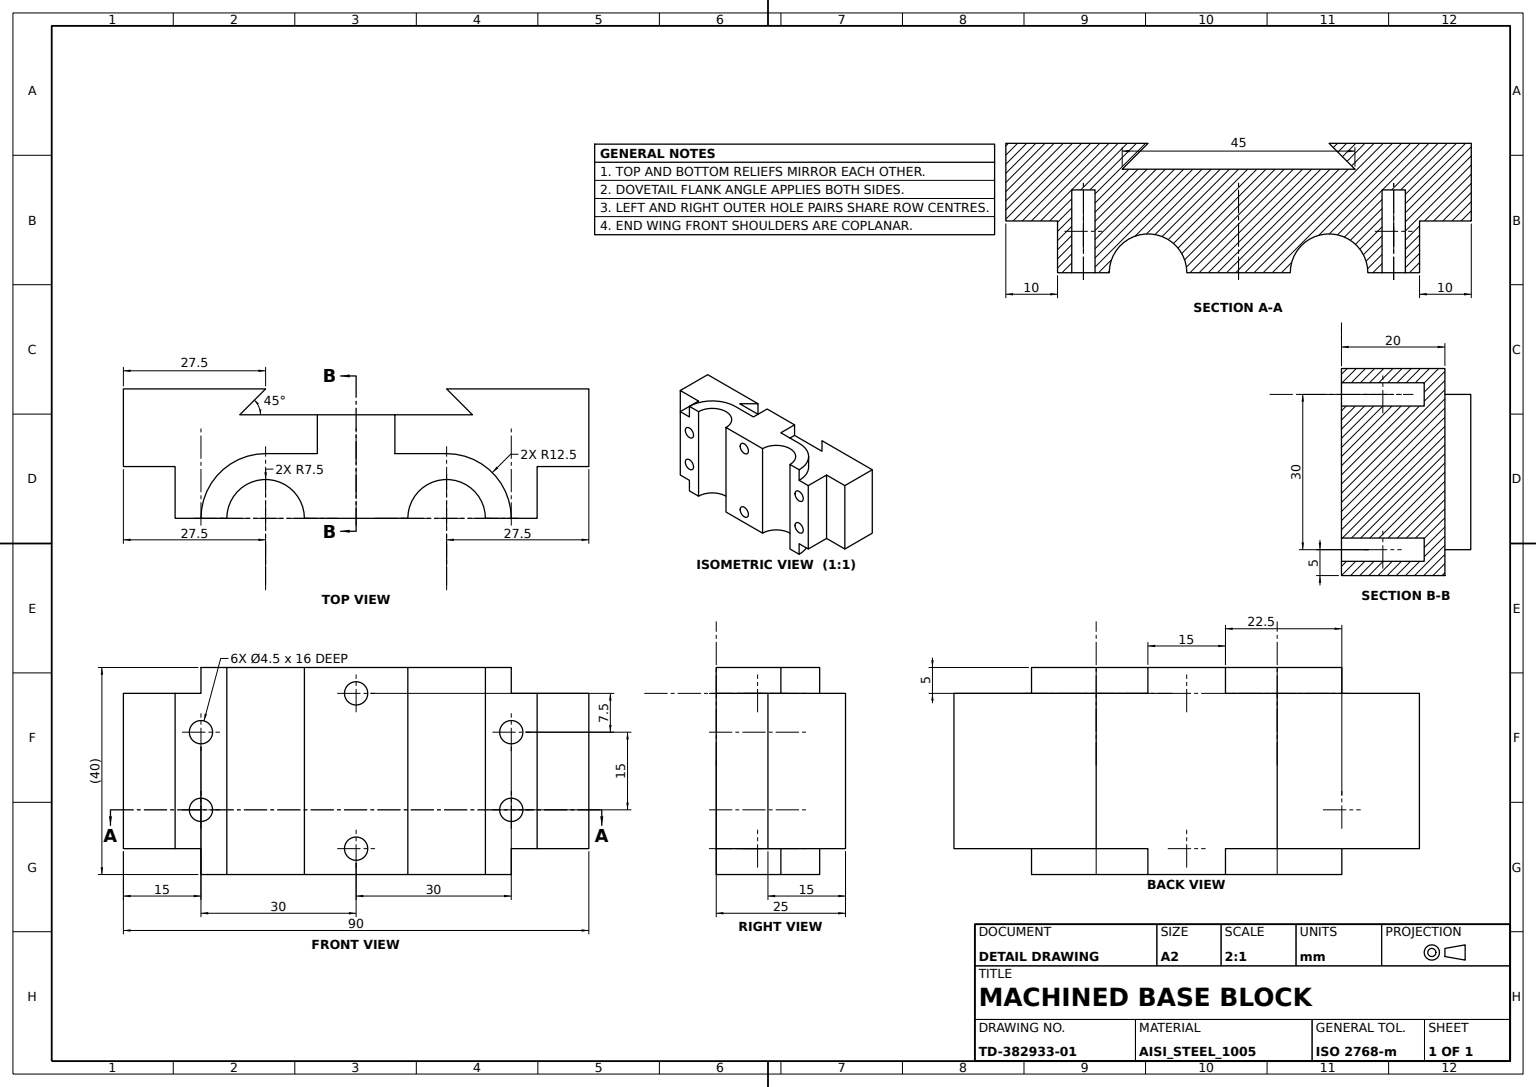
ISO-10303-21;
HEADER;
FILE_DESCRIPTION((''),'2;1');
FILE_NAME('','',(''),(''),'','','');
FILE_SCHEMA(('AUTOMOTIVE_DESIGN'));
ENDSEC;
DATA;
#1=APPLICATION_CONTEXT('');
#2=PRODUCT_CONTEXT('',#1,'mechanical');
#3=PRODUCT('','','',(#2));
#4=PRODUCT_DEFINITION_FORMATION('','',#3);
#5=PRODUCT_DEFINITION_CONTEXT('',#1,'design');
#6=PRODUCT_DEFINITION('','',#4,#5);
#7=PRODUCT_DEFINITION_SHAPE('','',#6);
#8=(LENGTH_UNIT()NAMED_UNIT(*)SI_UNIT(.MILLI.,.METRE.));
#9=(NAMED_UNIT(*)PLANE_ANGLE_UNIT()SI_UNIT($,.RADIAN.));
#10=(NAMED_UNIT(*)SI_UNIT($,.STERADIAN.)SOLID_ANGLE_UNIT());
#11=UNCERTAINTY_MEASURE_WITH_UNIT(LENGTH_MEASURE(0.005),#8,'distance_accuracy_value','');
#12=(GEOMETRIC_REPRESENTATION_CONTEXT(3)GLOBAL_UNCERTAINTY_ASSIGNED_CONTEXT((#11))GLOBAL_UNIT_ASSIGNED_CONTEXT((#8,#9,#10))REPRESENTATION_CONTEXT('',''));
#13=CARTESIAN_POINT('',(-20.,-27.75,-7.5));
#14=VERTEX_POINT('',#13);
#15=CARTESIAN_POINT('',(-20.,-30.,-7.5));
#16=DIRECTION('',(-1.,0.,0.));
#17=DIRECTION('',(0.,1.,0.));
#18=AXIS2_PLACEMENT_3D('',#15,#16,#17);
#19=CIRCLE('',#18,2.25);
#20=EDGE_CURVE('',#14,#14,#19,.T.);
#21=ORIENTED_EDGE('',*,*,#20,.T.);
#22=EDGE_LOOP('',(#21));
#23=FACE_BOUND('',#22,.T.);
#24=CARTESIAN_POINT('',(-4.,-27.75,-7.5));
#25=VERTEX_POINT('',#24);
#26=CARTESIAN_POINT('',(-4.,-30.,-7.5));
#27=AXIS2_PLACEMENT_3D('',#26,#16,#17);
#28=CIRCLE('',#27,2.25);
#29=EDGE_CURVE('',#25,#25,#28,.F.);
#30=ORIENTED_EDGE('',*,*,#29,.T.);
#31=EDGE_LOOP('',(#30));
#32=FACE_BOUND('',#31,.T.);
#33=DIRECTION('',(0.,0.,1.));
#34=AXIS2_PLACEMENT_3D('',#26,#16,#33);
#35=CYLINDRICAL_SURFACE('',#34,2.25);
#36=ADVANCED_FACE('',(#23,#32),#35,.F.);
#37=CARTESIAN_POINT('',(-4.,2.25,-15.));
#38=VERTEX_POINT('',#37);
#39=CARTESIAN_POINT('',(-4.,0.,-15.));
#40=AXIS2_PLACEMENT_3D('',#39,#16,#17);
#41=CIRCLE('',#40,2.25);
#42=EDGE_CURVE('',#38,#38,#41,.F.);
#43=ORIENTED_EDGE('',*,*,#42,.F.);
#44=EDGE_LOOP('',(#43));
#45=FACE_BOUND('',#44,.T.);
#46=AXIS2_PLACEMENT_3D('',#39,#16,#33);
#47=PLANE('',#46);
#48=ADVANCED_FACE('',(#45),#47,.T.);
#49=CARTESIAN_POINT('',(5.,17.5,15.));
#50=VERTEX_POINT('',#49);
#51=CARTESIAN_POINT('',(5.,17.5,-15.));
#52=VERTEX_POINT('',#51);
#53=DIRECTION('',(0.,0.,-1.));
#54=VECTOR('',#53,1000.);
#55=LINE('',#49,#54);
#56=EDGE_CURVE('',#50,#52,#55,.T.);
#57=ORIENTED_EDGE('',*,*,#56,.F.);
#58=CARTESIAN_POINT('',(0.,22.5,15.));
#59=VERTEX_POINT('',#58);
#60=DIRECTION('',(0.707106781,-0.707106781,0.));
#61=VECTOR('',#60,1000.);
#62=LINE('',#58,#61);
#63=EDGE_CURVE('',#59,#50,#62,.T.);
#64=ORIENTED_EDGE('',*,*,#63,.F.);
#65=CARTESIAN_POINT('',(0.,22.5,-15.));
#66=VERTEX_POINT('',#65);
#67=LINE('',#58,#54);
#68=EDGE_CURVE('',#59,#66,#67,.T.);
#69=ORIENTED_EDGE('',*,*,#68,.T.);
#70=LINE('',#65,#61);
#71=EDGE_CURVE('',#66,#52,#70,.T.);
#72=ORIENTED_EDGE('',*,*,#71,.T.);
#73=EDGE_LOOP('',(#57,#64,#69,#72));
#74=FACE_BOUND('',#73,.T.);
#75=DIRECTION('',(0.707106781,0.707106781,0.));
#76=DIRECTION('',(-0.707106781,0.707106781,0.));
#77=AXIS2_PLACEMENT_3D('',#58,#75,#76);
#78=PLANE('',#77);
#79=ADVANCED_FACE('',(#74),#78,.F.);
#80=CARTESIAN_POINT('',(-20.,2.25,-15.));
#81=VERTEX_POINT('',#80);
#82=CARTESIAN_POINT('',(-20.,0.,-15.));
#83=AXIS2_PLACEMENT_3D('',#82,#16,#17);
#84=CIRCLE('',#83,2.25);
#85=EDGE_CURVE('',#81,#81,#84,.T.);
#86=ORIENTED_EDGE('',*,*,#85,.T.);
#87=EDGE_LOOP('',(#86));
#88=FACE_BOUND('',#87,.T.);
#89=ORIENTED_EDGE('',*,*,#42,.T.);
#90=EDGE_LOOP('',(#89));
#91=FACE_BOUND('',#90,.T.);
#92=CYLINDRICAL_SURFACE('',#46,2.25);
#93=ADVANCED_FACE('',(#88,#91),#92,.F.);
#94=CARTESIAN_POINT('',(-4.,2.25,15.));
#95=VERTEX_POINT('',#94);
#96=CARTESIAN_POINT('',(-4.,0.,15.));
#97=AXIS2_PLACEMENT_3D('',#96,#16,#17);
#98=CIRCLE('',#97,2.25);
#99=EDGE_CURVE('',#95,#95,#98,.F.);
#100=ORIENTED_EDGE('',*,*,#99,.F.);
#101=EDGE_LOOP('',(#100));
#102=FACE_BOUND('',#101,.T.);
#103=AXIS2_PLACEMENT_3D('',#96,#16,#33);
#104=PLANE('',#103);
#105=ADVANCED_FACE('',(#102),#104,.T.);
#106=CARTESIAN_POINT('',(-20.,27.75,7.5));
#107=VERTEX_POINT('',#106);
#108=CARTESIAN_POINT('',(-20.,30.,7.5));
#109=DIRECTION('',(0.,-1.,0.));
#110=AXIS2_PLACEMENT_3D('',#108,#16,#109);
#111=CIRCLE('',#110,2.25);
#112=EDGE_CURVE('',#107,#107,#111,.T.);
#113=ORIENTED_EDGE('',*,*,#112,.T.);
#114=EDGE_LOOP('',(#113));
#115=FACE_BOUND('',#114,.T.);
#116=CARTESIAN_POINT('',(-4.,27.75,7.5));
#117=VERTEX_POINT('',#116);
#118=CARTESIAN_POINT('',(-4.,30.,7.5));
#119=AXIS2_PLACEMENT_3D('',#118,#16,#109);
#120=CIRCLE('',#119,2.25);
#121=EDGE_CURVE('',#117,#117,#120,.F.);
#122=ORIENTED_EDGE('',*,*,#121,.T.);
#123=EDGE_LOOP('',(#122));
#124=FACE_BOUND('',#123,.T.);
#125=AXIS2_PLACEMENT_3D('',#118,#16,#33);
#126=CYLINDRICAL_SURFACE('',#125,2.25);
#127=ADVANCED_FACE('',(#115,#124),#126,.F.);
#128=CARTESIAN_POINT('',(-20.,2.25,15.));
#129=VERTEX_POINT('',#128);
#130=CARTESIAN_POINT('',(-20.,0.,15.));
#131=AXIS2_PLACEMENT_3D('',#130,#16,#17);
#132=CIRCLE('',#131,2.25);
#133=EDGE_CURVE('',#129,#129,#132,.T.);
#134=ORIENTED_EDGE('',*,*,#133,.F.);
#135=EDGE_LOOP('',(#134));
#136=FACE_BOUND('',#135,.T.);
#137=ORIENTED_EDGE('',*,*,#85,.F.);
#138=EDGE_LOOP('',(#137));
#139=FACE_BOUND('',#138,.T.);
#140=CARTESIAN_POINT('',(-20.,10.,20.));
#141=VERTEX_POINT('',#140);
#142=CARTESIAN_POINT('',(-20.,10.,-20.));
#143=VERTEX_POINT('',#142);
#144=LINE('',#140,#54);
#145=EDGE_CURVE('',#141,#143,#144,.T.);
#146=ORIENTED_EDGE('',*,*,#145,.T.);
#147=CARTESIAN_POINT('',(-20.,-10.,-20.));
#148=VERTEX_POINT('',#147);
#149=VECTOR('',#109,1000.);
#150=LINE('',#142,#149);
#151=EDGE_CURVE('',#143,#148,#150,.T.);
#152=ORIENTED_EDGE('',*,*,#151,.T.);
#153=CARTESIAN_POINT('',(-20.,-10.,20.));
#154=VERTEX_POINT('',#153);
#155=LINE('',#153,#54);
#156=EDGE_CURVE('',#154,#148,#155,.T.);
#157=ORIENTED_EDGE('',*,*,#156,.F.);
#158=LINE('',#140,#149);
#159=EDGE_CURVE('',#141,#154,#158,.T.);
#160=ORIENTED_EDGE('',*,*,#159,.F.);
#161=EDGE_LOOP('',(#146,#152,#157,#160));
#162=FACE_BOUND('',#161,.T.);
#163=DIRECTION('',(1.,0.,0.));
#164=AXIS2_PLACEMENT_3D('',#140,#163,#53);
#165=PLANE('',#164);
#166=ADVANCED_FACE('',(#136,#139,#162),#165,.F.);
#167=CARTESIAN_POINT('',(5.,-17.5,-15.));
#168=VERTEX_POINT('',#167);
#169=CARTESIAN_POINT('',(0.,-22.5,-15.));
#170=VERTEX_POINT('',#169);
#171=DIRECTION('',(-0.707106781,-0.707106781,0.));
#172=VECTOR('',#171,1000.);
#173=LINE('',#167,#172);
#174=EDGE_CURVE('',#168,#170,#173,.T.);
#175=ORIENTED_EDGE('',*,*,#174,.T.);
#176=CARTESIAN_POINT('',(0.,-22.5,15.));
#177=VERTEX_POINT('',#176);
#178=LINE('',#176,#54);
#179=EDGE_CURVE('',#177,#170,#178,.T.);
#180=ORIENTED_EDGE('',*,*,#179,.F.);
#181=CARTESIAN_POINT('',(5.,-17.5,15.));
#182=VERTEX_POINT('',#181);
#183=LINE('',#181,#172);
#184=EDGE_CURVE('',#182,#177,#183,.T.);
#185=ORIENTED_EDGE('',*,*,#184,.F.);
#186=LINE('',#181,#54);
#187=EDGE_CURVE('',#182,#168,#186,.T.);
#188=ORIENTED_EDGE('',*,*,#187,.T.);
#189=EDGE_LOOP('',(#175,#180,#185,#188));
#190=FACE_BOUND('',#189,.T.);
#191=AXIS2_PLACEMENT_3D('',#181,#60,#75);
#192=PLANE('',#191);
#193=ADVANCED_FACE('',(#190),#192,.F.);
#194=CARTESIAN_POINT('',(-20.,-30.,15.));
#195=VERTEX_POINT('',#194);
#196=CARTESIAN_POINT('',(-20.,-35.,15.));
#197=VERTEX_POINT('',#196);
#198=LINE('',#194,#149);
#199=EDGE_CURVE('',#195,#197,#198,.T.);
#200=ORIENTED_EDGE('',*,*,#199,.T.);
#201=CARTESIAN_POINT('',(-10.,-35.,15.));
#202=VERTEX_POINT('',#201);
#203=VECTOR('',#163,1000.);
#204=LINE('',#196,#203);
#205=EDGE_CURVE('',#197,#202,#204,.T.);
#206=ORIENTED_EDGE('',*,*,#205,.T.);
#207=CARTESIAN_POINT('',(-10.,-45.,15.));
#208=VERTEX_POINT('',#207);
#209=LINE('',#201,#149);
#210=EDGE_CURVE('',#202,#208,#209,.T.);
#211=ORIENTED_EDGE('',*,*,#210,.T.);
#212=CARTESIAN_POINT('',(5.,-45.,15.));
#213=VERTEX_POINT('',#212);
#214=LINE('',#207,#203);
#215=EDGE_CURVE('',#208,#213,#214,.T.);
#216=ORIENTED_EDGE('',*,*,#215,.T.);
#217=VECTOR('',#17,1000.);
#218=LINE('',#212,#217);
#219=EDGE_CURVE('',#213,#182,#218,.T.);
#220=ORIENTED_EDGE('',*,*,#219,.T.);
#221=ORIENTED_EDGE('',*,*,#184,.T.);
#222=CARTESIAN_POINT('',(0.,-7.5,15.));
#223=VERTEX_POINT('',#222);
#224=LINE('',#176,#217);
#225=EDGE_CURVE('',#177,#223,#224,.T.);
#226=ORIENTED_EDGE('',*,*,#225,.T.);
#227=CARTESIAN_POINT('',(-7.5,-7.5,15.));
#228=VERTEX_POINT('',#227);
#229=VECTOR('',#16,1000.);
#230=LINE('',#222,#229);
#231=EDGE_CURVE('',#223,#228,#230,.T.);
#232=ORIENTED_EDGE('',*,*,#231,.T.);
#233=CARTESIAN_POINT('',(-7.5,-17.5,15.));
#234=VERTEX_POINT('',#233);
#235=LINE('',#227,#149);
#236=EDGE_CURVE('',#228,#234,#235,.T.);
#237=ORIENTED_EDGE('',*,*,#236,.T.);
#238=CARTESIAN_POINT('',(-20.,-17.5,15.));
#239=AXIS2_PLACEMENT_3D('',#238,#53,#17);
#240=CIRCLE('',#239,12.5);
#241=EDGE_CURVE('',#234,#195,#240,.T.);
#242=ORIENTED_EDGE('',*,*,#241,.T.);
#243=EDGE_LOOP('',(#200,#206,#211,#216,#220,#221,#226,#232,#237,#242));
#244=FACE_BOUND('',#243,.T.);
#245=AXIS2_PLACEMENT_3D('',#238,#53,#16);
#246=PLANE('',#245);
#247=ADVANCED_FACE('',(#244),#246,.F.);
#248=CARTESIAN_POINT('',(-7.5,-17.5,20.));
#249=VERTEX_POINT('',#248);
#250=LINE('',#248,#54);
#251=EDGE_CURVE('',#249,#234,#250,.T.);
#252=ORIENTED_EDGE('',*,*,#251,.F.);
#253=CARTESIAN_POINT('',(-20.,-30.,20.));
#254=VERTEX_POINT('',#253);
#255=CARTESIAN_POINT('',(-20.,-17.5,20.));
#256=AXIS2_PLACEMENT_3D('',#255,#33,#17);
#257=CIRCLE('',#256,12.5);
#258=EDGE_CURVE('',#254,#249,#257,.T.);
#259=ORIENTED_EDGE('',*,*,#258,.F.);
#260=LINE('',#253,#54);
#261=EDGE_CURVE('',#254,#195,#260,.T.);
#262=ORIENTED_EDGE('',*,*,#261,.T.);
#263=ORIENTED_EDGE('',*,*,#241,.F.);
#264=EDGE_LOOP('',(#252,#259,#262,#263));
#265=FACE_BOUND('',#264,.T.);
#266=AXIS2_PLACEMENT_3D('',#255,#53,#16);
#267=CYLINDRICAL_SURFACE('',#266,12.5);
#268=ADVANCED_FACE('',(#265),#267,.T.);
#269=CARTESIAN_POINT('',(-10.,45.,15.));
#270=VERTEX_POINT('',#269);
#271=CARTESIAN_POINT('',(-10.,35.,15.));
#272=VERTEX_POINT('',#271);
#273=LINE('',#269,#149);
#274=EDGE_CURVE('',#270,#272,#273,.T.);
#275=ORIENTED_EDGE('',*,*,#274,.T.);
#276=CARTESIAN_POINT('',(-20.,35.,15.));
#277=VERTEX_POINT('',#276);
#278=LINE('',#271,#229);
#279=EDGE_CURVE('',#272,#277,#278,.T.);
#280=ORIENTED_EDGE('',*,*,#279,.T.);
#281=CARTESIAN_POINT('',(-20.,30.,15.));
#282=VERTEX_POINT('',#281);
#283=LINE('',#276,#149);
#284=EDGE_CURVE('',#277,#282,#283,.T.);
#285=ORIENTED_EDGE('',*,*,#284,.T.);
#286=CARTESIAN_POINT('',(-7.5,17.5,15.));
#287=VERTEX_POINT('',#286);
#288=CARTESIAN_POINT('',(-20.,17.5,15.));
#289=AXIS2_PLACEMENT_3D('',#288,#53,#109);
#290=CIRCLE('',#289,12.5);
#291=EDGE_CURVE('',#282,#287,#290,.T.);
#292=ORIENTED_EDGE('',*,*,#291,.T.);
#293=CARTESIAN_POINT('',(-7.5,7.5,15.));
#294=VERTEX_POINT('',#293);
#295=LINE('',#286,#149);
#296=EDGE_CURVE('',#287,#294,#295,.T.);
#297=ORIENTED_EDGE('',*,*,#296,.T.);
#298=CARTESIAN_POINT('',(0.,7.5,15.));
#299=VERTEX_POINT('',#298);
#300=LINE('',#293,#203);
#301=EDGE_CURVE('',#294,#299,#300,.T.);
#302=ORIENTED_EDGE('',*,*,#301,.T.);
#303=LINE('',#298,#217);
#304=EDGE_CURVE('',#299,#59,#303,.T.);
#305=ORIENTED_EDGE('',*,*,#304,.T.);
#306=ORIENTED_EDGE('',*,*,#63,.T.);
#307=CARTESIAN_POINT('',(5.,45.,15.));
#308=VERTEX_POINT('',#307);
#309=LINE('',#49,#217);
#310=EDGE_CURVE('',#50,#308,#309,.T.);
#311=ORIENTED_EDGE('',*,*,#310,.T.);
#312=LINE('',#307,#229);
#313=EDGE_CURVE('',#308,#270,#312,.T.);
#314=ORIENTED_EDGE('',*,*,#313,.T.);
#315=EDGE_LOOP('',(#275,#280,#285,#292,#297,#302,#305,#306,#311,#314));
#316=FACE_BOUND('',#315,.T.);
#317=AXIS2_PLACEMENT_3D('',#288,#53,#16);
#318=PLANE('',#317);
#319=ADVANCED_FACE('',(#316),#318,.F.);
#320=CARTESIAN_POINT('',(0.,-7.5,-15.));
#321=VERTEX_POINT('',#320);
#322=CARTESIAN_POINT('',(-7.5,-7.5,-15.));
#323=VERTEX_POINT('',#322);
#324=LINE('',#320,#229);
#325=EDGE_CURVE('',#321,#323,#324,.T.);
#326=ORIENTED_EDGE('',*,*,#325,.T.);
#327=CARTESIAN_POINT('',(-7.5,-7.5,-20.));
#328=VERTEX_POINT('',#327);
#329=CARTESIAN_POINT('',(-7.5,-7.5,20.));
#330=LINE('',#329,#54);
#331=EDGE_CURVE('',#323,#328,#330,.T.);
#332=ORIENTED_EDGE('',*,*,#331,.T.);
#333=CARTESIAN_POINT('',(0.,-7.5,-20.));
#334=VERTEX_POINT('',#333);
#335=LINE('',#327,#203);
#336=EDGE_CURVE('',#328,#334,#335,.T.);
#337=ORIENTED_EDGE('',*,*,#336,.T.);
#338=CARTESIAN_POINT('',(0.,-7.5,20.));
#339=LINE('',#338,#54);
#340=EDGE_CURVE('',#321,#334,#339,.T.);
#341=ORIENTED_EDGE('',*,*,#340,.F.);
#342=EDGE_LOOP('',(#326,#332,#337,#341));
#343=FACE_BOUND('',#342,.T.);
#344=AXIS2_PLACEMENT_3D('',#329,#17,#16);
#345=PLANE('',#344);
#346=ADVANCED_FACE('',(#343),#345,.F.);
#347=CARTESIAN_POINT('',(-20.,27.75,-7.5));
#348=VERTEX_POINT('',#347);
#349=CARTESIAN_POINT('',(-20.,30.,-7.5));
#350=AXIS2_PLACEMENT_3D('',#349,#16,#109);
#351=CIRCLE('',#350,2.25);
#352=EDGE_CURVE('',#348,#348,#351,.T.);
#353=ORIENTED_EDGE('',*,*,#352,.F.);
#354=EDGE_LOOP('',(#353));
#355=FACE_BOUND('',#354,.T.);
#356=ORIENTED_EDGE('',*,*,#284,.F.);
#357=CARTESIAN_POINT('',(-20.,35.,-15.));
#358=VERTEX_POINT('',#357);
#359=LINE('',#276,#54);
#360=EDGE_CURVE('',#277,#358,#359,.T.);
#361=ORIENTED_EDGE('',*,*,#360,.T.);
#362=CARTESIAN_POINT('',(-20.,30.,-15.));
#363=VERTEX_POINT('',#362);
#364=LINE('',#357,#149);
#365=EDGE_CURVE('',#358,#363,#364,.T.);
#366=ORIENTED_EDGE('',*,*,#365,.T.);
#367=CARTESIAN_POINT('',(-20.,30.,-20.));
#368=VERTEX_POINT('',#367);
#369=CARTESIAN_POINT('',(-20.,30.,20.));
#370=LINE('',#369,#54);
#371=EDGE_CURVE('',#363,#368,#370,.T.);
#372=ORIENTED_EDGE('',*,*,#371,.T.);
#373=CARTESIAN_POINT('',(-20.,25.,-20.));
#374=VERTEX_POINT('',#373);
#375=LINE('',#367,#149);
#376=EDGE_CURVE('',#368,#374,#375,.T.);
#377=ORIENTED_EDGE('',*,*,#376,.T.);
#378=CARTESIAN_POINT('',(-20.,25.,20.));
#379=VERTEX_POINT('',#378);
#380=LINE('',#378,#54);
#381=EDGE_CURVE('',#379,#374,#380,.T.);
#382=ORIENTED_EDGE('',*,*,#381,.F.);
#383=VERTEX_POINT('',#369);
#384=LINE('',#369,#149);
#385=EDGE_CURVE('',#383,#379,#384,.T.);
#386=ORIENTED_EDGE('',*,*,#385,.F.);
#387=EDGE_CURVE('',#383,#282,#370,.T.);
#388=ORIENTED_EDGE('',*,*,#387,.T.);
#389=EDGE_LOOP('',(#356,#361,#366,#372,#377,#382,#386,#388));
#390=FACE_BOUND('',#389,.T.);
#391=ORIENTED_EDGE('',*,*,#112,.F.);
#392=EDGE_LOOP('',(#391));
#393=FACE_BOUND('',#392,.T.);
#394=AXIS2_PLACEMENT_3D('',#369,#163,#53);
#395=PLANE('',#394);
#396=ADVANCED_FACE('',(#355,#390,#393),#395,.F.);
#397=CARTESIAN_POINT('',(-20.,-25.,-20.));
#398=VERTEX_POINT('',#397);
#399=CARTESIAN_POINT('',(-20.,-17.5,-20.));
#400=AXIS2_PLACEMENT_3D('',#399,#53,#17);
#401=CIRCLE('',#400,7.5);
#402=EDGE_CURVE('',#148,#398,#401,.T.);
#403=ORIENTED_EDGE('',*,*,#402,.T.);
#404=CARTESIAN_POINT('',(-20.,-25.,20.));
#405=VERTEX_POINT('',#404);
#406=LINE('',#404,#54);
#407=EDGE_CURVE('',#405,#398,#406,.T.);
#408=ORIENTED_EDGE('',*,*,#407,.F.);
#409=AXIS2_PLACEMENT_3D('',#255,#53,#17);
#410=CIRCLE('',#409,7.5);
#411=EDGE_CURVE('',#154,#405,#410,.T.);
#412=ORIENTED_EDGE('',*,*,#411,.F.);
#413=ORIENTED_EDGE('',*,*,#156,.T.);
#414=EDGE_LOOP('',(#403,#408,#412,#413));
#415=FACE_BOUND('',#414,.T.);
#416=CYLINDRICAL_SURFACE('',#266,7.5);
#417=ADVANCED_FACE('',(#415),#416,.F.);
#418=CARTESIAN_POINT('',(-4.,-27.75,7.5));
#419=VERTEX_POINT('',#418);
#420=CARTESIAN_POINT('',(-4.,-30.,7.5));
#421=AXIS2_PLACEMENT_3D('',#420,#16,#17);
#422=CIRCLE('',#421,2.25);
#423=EDGE_CURVE('',#419,#419,#422,.F.);
#424=ORIENTED_EDGE('',*,*,#423,.F.);
#425=EDGE_LOOP('',(#424));
#426=FACE_BOUND('',#425,.T.);
#427=AXIS2_PLACEMENT_3D('',#420,#16,#33);
#428=PLANE('',#427);
#429=ADVANCED_FACE('',(#426),#428,.T.);
#430=CARTESIAN_POINT('',(-7.5,7.5,20.));
#431=VERTEX_POINT('',#430);
#432=LINE('',#430,#54);
#433=EDGE_CURVE('',#431,#294,#432,.T.);
#434=ORIENTED_EDGE('',*,*,#433,.T.);
#435=ORIENTED_EDGE('',*,*,#296,.F.);
#436=CARTESIAN_POINT('',(-7.5,17.5,20.));
#437=VERTEX_POINT('',#436);
#438=LINE('',#436,#54);
#439=EDGE_CURVE('',#437,#287,#438,.T.);
#440=ORIENTED_EDGE('',*,*,#439,.F.);
#441=LINE('',#430,#217);
#442=EDGE_CURVE('',#431,#437,#441,.T.);
#443=ORIENTED_EDGE('',*,*,#442,.F.);
#444=EDGE_LOOP('',(#434,#435,#440,#443));
#445=FACE_BOUND('',#444,.T.);
#446=AXIS2_PLACEMENT_3D('',#430,#16,#109);
#447=PLANE('',#446);
#448=ADVANCED_FACE('',(#445),#447,.F.);
#449=CARTESIAN_POINT('',(-10.,-35.,-15.));
#450=VERTEX_POINT('',#449);
#451=LINE('',#201,#54);
#452=EDGE_CURVE('',#202,#450,#451,.T.);
#453=ORIENTED_EDGE('',*,*,#452,.F.);
#454=ORIENTED_EDGE('',*,*,#205,.F.);
#455=CARTESIAN_POINT('',(-20.,-35.,-15.));
#456=VERTEX_POINT('',#455);
#457=LINE('',#196,#54);
#458=EDGE_CURVE('',#197,#456,#457,.T.);
#459=ORIENTED_EDGE('',*,*,#458,.T.);
#460=LINE('',#455,#203);
#461=EDGE_CURVE('',#456,#450,#460,.T.);
#462=ORIENTED_EDGE('',*,*,#461,.T.);
#463=EDGE_LOOP('',(#453,#454,#459,#462));
#464=FACE_BOUND('',#463,.T.);
#465=AXIS2_PLACEMENT_3D('',#196,#17,#33);
#466=PLANE('',#465);
#467=ADVANCED_FACE('',(#464),#466,.F.);
#468=CARTESIAN_POINT('',(0.,7.5,-15.));
#469=VERTEX_POINT('',#468);
#470=LINE('',#468,#217);
#471=EDGE_CURVE('',#469,#66,#470,.T.);
#472=ORIENTED_EDGE('',*,*,#471,.T.);
#473=ORIENTED_EDGE('',*,*,#68,.F.);
#474=ORIENTED_EDGE('',*,*,#304,.F.);
#475=CARTESIAN_POINT('',(0.,7.5,20.));
#476=VERTEX_POINT('',#475);
#477=LINE('',#475,#54);
#478=EDGE_CURVE('',#476,#299,#477,.T.);
#479=ORIENTED_EDGE('',*,*,#478,.F.);
#480=VERTEX_POINT('',#338);
#481=LINE('',#338,#217);
#482=EDGE_CURVE('',#480,#476,#481,.T.);
#483=ORIENTED_EDGE('',*,*,#482,.F.);
#484=EDGE_CURVE('',#480,#223,#339,.T.);
#485=ORIENTED_EDGE('',*,*,#484,.T.);
#486=ORIENTED_EDGE('',*,*,#225,.F.);
#487=ORIENTED_EDGE('',*,*,#179,.T.);
#488=LINE('',#169,#217);
#489=EDGE_CURVE('',#170,#321,#488,.T.);
#490=ORIENTED_EDGE('',*,*,#489,.T.);
#491=ORIENTED_EDGE('',*,*,#340,.T.);
#492=CARTESIAN_POINT('',(0.,7.5,-20.));
#493=VERTEX_POINT('',#492);
#494=LINE('',#333,#217);
#495=EDGE_CURVE('',#334,#493,#494,.T.);
#496=ORIENTED_EDGE('',*,*,#495,.T.);
#497=EDGE_CURVE('',#469,#493,#477,.T.);
#498=ORIENTED_EDGE('',*,*,#497,.F.);
#499=EDGE_LOOP('',(#472,#473,#474,#479,#483,#485,#486,#487,#490,#491,#496,#498));
#500=FACE_BOUND('',#499,.T.);
#501=AXIS2_PLACEMENT_3D('',#338,#16,#33);
#502=PLANE('',#501);
#503=ADVANCED_FACE('',(#500),#502,.F.);
#504=CARTESIAN_POINT('',(-20.,-27.75,7.5));
#505=VERTEX_POINT('',#504);
#506=CARTESIAN_POINT('',(-20.,-30.,7.5));
#507=AXIS2_PLACEMENT_3D('',#506,#16,#17);
#508=CIRCLE('',#507,2.25);
#509=EDGE_CURVE('',#505,#505,#508,.T.);
#510=ORIENTED_EDGE('',*,*,#509,.T.);
#511=EDGE_LOOP('',(#510));
#512=FACE_BOUND('',#511,.T.);
#513=ORIENTED_EDGE('',*,*,#423,.T.);
#514=EDGE_LOOP('',(#513));
#515=FACE_BOUND('',#514,.T.);
#516=CYLINDRICAL_SURFACE('',#427,2.25);
#517=ADVANCED_FACE('',(#512,#515),#516,.F.);
#518=CARTESIAN_POINT('',(-4.,27.75,-7.5));
#519=VERTEX_POINT('',#518);
#520=CARTESIAN_POINT('',(-4.,30.,-7.5));
#521=AXIS2_PLACEMENT_3D('',#520,#16,#109);
#522=CIRCLE('',#521,2.25);
#523=EDGE_CURVE('',#519,#519,#522,.F.);
#524=ORIENTED_EDGE('',*,*,#523,.T.);
#525=EDGE_LOOP('',(#524));
#526=FACE_BOUND('',#525,.T.);
#527=ORIENTED_EDGE('',*,*,#352,.T.);
#528=EDGE_LOOP('',(#527));
#529=FACE_BOUND('',#528,.T.);
#530=AXIS2_PLACEMENT_3D('',#520,#16,#33);
#531=CYLINDRICAL_SURFACE('',#530,2.25);
#532=ADVANCED_FACE('',(#526,#529),#531,.F.);
#533=ORIENTED_EDGE('',*,*,#325,.F.);
#534=ORIENTED_EDGE('',*,*,#489,.F.);
#535=ORIENTED_EDGE('',*,*,#174,.F.);
#536=CARTESIAN_POINT('',(5.,-45.,-15.));
#537=VERTEX_POINT('',#536);
#538=LINE('',#536,#217);
#539=EDGE_CURVE('',#537,#168,#538,.T.);
#540=ORIENTED_EDGE('',*,*,#539,.F.);
#541=CARTESIAN_POINT('',(-10.,-45.,-15.));
#542=VERTEX_POINT('',#541);
#543=LINE('',#541,#203);
#544=EDGE_CURVE('',#542,#537,#543,.T.);
#545=ORIENTED_EDGE('',*,*,#544,.F.);
#546=LINE('',#449,#149);
#547=EDGE_CURVE('',#450,#542,#546,.T.);
#548=ORIENTED_EDGE('',*,*,#547,.F.);
#549=ORIENTED_EDGE('',*,*,#461,.F.);
#550=CARTESIAN_POINT('',(-20.,-30.,-15.));
#551=VERTEX_POINT('',#550);
#552=LINE('',#550,#149);
#553=EDGE_CURVE('',#551,#456,#552,.T.);
#554=ORIENTED_EDGE('',*,*,#553,.F.);
#555=CARTESIAN_POINT('',(-7.5,-17.5,-15.));
#556=VERTEX_POINT('',#555);
#557=CARTESIAN_POINT('',(-20.,-17.5,-15.));
#558=AXIS2_PLACEMENT_3D('',#557,#53,#17);
#559=CIRCLE('',#558,12.5);
#560=EDGE_CURVE('',#556,#551,#559,.T.);
#561=ORIENTED_EDGE('',*,*,#560,.F.);
#562=LINE('',#322,#149);
#563=EDGE_CURVE('',#323,#556,#562,.T.);
#564=ORIENTED_EDGE('',*,*,#563,.F.);
#565=EDGE_LOOP('',(#533,#534,#535,#540,#545,#548,#549,#554,#561,#564));
#566=FACE_BOUND('',#565,.T.);
#567=AXIS2_PLACEMENT_3D('',#557,#53,#16);
#568=PLANE('',#567);
#569=ADVANCED_FACE('',(#566),#568,.T.);
#570=ORIENTED_EDGE('',*,*,#452,.T.);
#571=ORIENTED_EDGE('',*,*,#547,.T.);
#572=LINE('',#207,#54);
#573=EDGE_CURVE('',#208,#542,#572,.T.);
#574=ORIENTED_EDGE('',*,*,#573,.F.);
#575=ORIENTED_EDGE('',*,*,#210,.F.);
#576=EDGE_LOOP('',(#570,#571,#574,#575));
#577=FACE_BOUND('',#576,.T.);
#578=AXIS2_PLACEMENT_3D('',#201,#163,#17);
#579=PLANE('',#578);
#580=ADVANCED_FACE('',(#577),#579,.F.);
#581=ORIENTED_EDGE('',*,*,#231,.F.);
#582=ORIENTED_EDGE('',*,*,#484,.F.);
#583=VERTEX_POINT('',#329);
#584=LINE('',#329,#203);
#585=EDGE_CURVE('',#583,#480,#584,.T.);
#586=ORIENTED_EDGE('',*,*,#585,.F.);
#587=EDGE_CURVE('',#583,#228,#330,.T.);
#588=ORIENTED_EDGE('',*,*,#587,.T.);
#589=EDGE_LOOP('',(#581,#582,#586,#588));
#590=FACE_BOUND('',#589,.T.);
#591=ADVANCED_FACE('',(#590),#345,.F.);
#592=ORIENTED_EDGE('',*,*,#219,.F.);
#593=LINE('',#212,#54);
#594=EDGE_CURVE('',#213,#537,#593,.T.);
#595=ORIENTED_EDGE('',*,*,#594,.T.);
#596=ORIENTED_EDGE('',*,*,#539,.T.);
#597=ORIENTED_EDGE('',*,*,#187,.F.);
#598=EDGE_LOOP('',(#592,#595,#596,#597));
#599=FACE_BOUND('',#598,.T.);
#600=AXIS2_PLACEMENT_3D('',#212,#16,#33);
#601=PLANE('',#600);
#602=ADVANCED_FACE('',(#599),#601,.F.);
#603=CARTESIAN_POINT('',(-20.,17.5,20.));
#604=AXIS2_PLACEMENT_3D('',#603,#53,#109);
#605=CIRCLE('',#604,7.5);
#606=EDGE_CURVE('',#379,#141,#605,.T.);
#607=ORIENTED_EDGE('',*,*,#606,.T.);
#608=ORIENTED_EDGE('',*,*,#159,.T.);
#609=ORIENTED_EDGE('',*,*,#411,.T.);
#610=LINE('',#404,#149);
#611=EDGE_CURVE('',#405,#254,#610,.T.);
#612=ORIENTED_EDGE('',*,*,#611,.T.);
#613=ORIENTED_EDGE('',*,*,#258,.T.);
#614=LINE('',#248,#217);
#615=EDGE_CURVE('',#249,#583,#614,.T.);
#616=ORIENTED_EDGE('',*,*,#615,.T.);
#617=ORIENTED_EDGE('',*,*,#585,.T.);
#618=ORIENTED_EDGE('',*,*,#482,.T.);
#619=LINE('',#475,#229);
#620=EDGE_CURVE('',#476,#431,#619,.T.);
#621=ORIENTED_EDGE('',*,*,#620,.T.);
#622=ORIENTED_EDGE('',*,*,#442,.T.);
#623=AXIS2_PLACEMENT_3D('',#603,#33,#109);
#624=CIRCLE('',#623,12.5);
#625=EDGE_CURVE('',#437,#383,#624,.T.);
#626=ORIENTED_EDGE('',*,*,#625,.T.);
#627=ORIENTED_EDGE('',*,*,#385,.T.);
#628=EDGE_LOOP('',(#607,#608,#609,#612,#613,#616,#617,#618,#621,#622,#626,#627));
#629=FACE_BOUND('',#628,.T.);
#630=AXIS2_PLACEMENT_3D('',#255,#33,#163);
#631=PLANE('',#630);
#632=ADVANCED_FACE('',(#629),#631,.T.);
#633=ORIENTED_EDGE('',*,*,#573,.T.);
#634=ORIENTED_EDGE('',*,*,#544,.T.);
#635=ORIENTED_EDGE('',*,*,#594,.F.);
#636=ORIENTED_EDGE('',*,*,#215,.F.);
#637=EDGE_LOOP('',(#633,#634,#635,#636));
#638=FACE_BOUND('',#637,.T.);
#639=AXIS2_PLACEMENT_3D('',#207,#17,#33);
#640=PLANE('',#639);
#641=ADVANCED_FACE('',(#638),#640,.F.);
#642=CARTESIAN_POINT('',(-10.,45.,-15.));
#643=VERTEX_POINT('',#642);
#644=CARTESIAN_POINT('',(-10.,35.,-15.));
#645=VERTEX_POINT('',#644);
#646=LINE('',#642,#149);
#647=EDGE_CURVE('',#643,#645,#646,.T.);
#648=ORIENTED_EDGE('',*,*,#647,.F.);
#649=CARTESIAN_POINT('',(5.,45.,-15.));
#650=VERTEX_POINT('',#649);
#651=LINE('',#649,#229);
#652=EDGE_CURVE('',#650,#643,#651,.T.);
#653=ORIENTED_EDGE('',*,*,#652,.F.);
#654=LINE('',#51,#217);
#655=EDGE_CURVE('',#52,#650,#654,.T.);
#656=ORIENTED_EDGE('',*,*,#655,.F.);
#657=ORIENTED_EDGE('',*,*,#71,.F.);
#658=ORIENTED_EDGE('',*,*,#471,.F.);
#659=CARTESIAN_POINT('',(-7.5,7.5,-15.));
#660=VERTEX_POINT('',#659);
#661=LINE('',#659,#203);
#662=EDGE_CURVE('',#660,#469,#661,.T.);
#663=ORIENTED_EDGE('',*,*,#662,.F.);
#664=CARTESIAN_POINT('',(-7.5,17.5,-15.));
#665=VERTEX_POINT('',#664);
#666=LINE('',#664,#149);
#667=EDGE_CURVE('',#665,#660,#666,.T.);
#668=ORIENTED_EDGE('',*,*,#667,.F.);
#669=CARTESIAN_POINT('',(-20.,17.5,-15.));
#670=AXIS2_PLACEMENT_3D('',#669,#53,#109);
#671=CIRCLE('',#670,12.5);
#672=EDGE_CURVE('',#363,#665,#671,.T.);
#673=ORIENTED_EDGE('',*,*,#672,.F.);
#674=ORIENTED_EDGE('',*,*,#365,.F.);
#675=LINE('',#644,#229);
#676=EDGE_CURVE('',#645,#358,#675,.T.);
#677=ORIENTED_EDGE('',*,*,#676,.F.);
#678=EDGE_LOOP('',(#648,#653,#656,#657,#658,#663,#668,#673,#674,#677));
#679=FACE_BOUND('',#678,.T.);
#680=AXIS2_PLACEMENT_3D('',#669,#53,#16);
#681=PLANE('',#680);
#682=ADVANCED_FACE('',(#679),#681,.T.);
#683=ORIENTED_EDGE('',*,*,#647,.T.);
#684=LINE('',#271,#54);
#685=EDGE_CURVE('',#272,#645,#684,.T.);
#686=ORIENTED_EDGE('',*,*,#685,.F.);
#687=ORIENTED_EDGE('',*,*,#274,.F.);
#688=LINE('',#269,#54);
#689=EDGE_CURVE('',#270,#643,#688,.T.);
#690=ORIENTED_EDGE('',*,*,#689,.T.);
#691=EDGE_LOOP('',(#683,#686,#687,#690));
#692=FACE_BOUND('',#691,.T.);
#693=AXIS2_PLACEMENT_3D('',#269,#163,#17);
#694=PLANE('',#693);
#695=ADVANCED_FACE('',(#692),#694,.F.);
#696=CARTESIAN_POINT('',(-20.,-30.,-20.));
#697=VERTEX_POINT('',#696);
#698=CARTESIAN_POINT('',(-7.5,-17.5,-20.));
#699=VERTEX_POINT('',#698);
#700=AXIS2_PLACEMENT_3D('',#399,#33,#17);
#701=CIRCLE('',#700,12.5);
#702=EDGE_CURVE('',#697,#699,#701,.T.);
#703=ORIENTED_EDGE('',*,*,#702,.T.);
#704=EDGE_CURVE('',#556,#699,#250,.T.);
#705=ORIENTED_EDGE('',*,*,#704,.F.);
#706=ORIENTED_EDGE('',*,*,#560,.T.);
#707=EDGE_CURVE('',#551,#697,#260,.T.);
#708=ORIENTED_EDGE('',*,*,#707,.T.);
#709=EDGE_LOOP('',(#703,#705,#706,#708));
#710=FACE_BOUND('',#709,.T.);
#711=ADVANCED_FACE('',(#710),#267,.T.);
#712=ORIENTED_EDGE('',*,*,#29,.F.);
#713=EDGE_LOOP('',(#712));
#714=FACE_BOUND('',#713,.T.);
#715=PLANE('',#34);
#716=ADVANCED_FACE('',(#714),#715,.T.);
#717=ORIENTED_EDGE('',*,*,#236,.F.);
#718=ORIENTED_EDGE('',*,*,#587,.F.);
#719=ORIENTED_EDGE('',*,*,#615,.F.);
#720=ORIENTED_EDGE('',*,*,#251,.T.);
#721=EDGE_LOOP('',(#717,#718,#719,#720));
#722=FACE_BOUND('',#721,.T.);
#723=AXIS2_PLACEMENT_3D('',#248,#16,#109);
#724=PLANE('',#723);
#725=ADVANCED_FACE('',(#722),#724,.F.);
#726=ORIENTED_EDGE('',*,*,#56,.T.);
#727=ORIENTED_EDGE('',*,*,#655,.T.);
#728=LINE('',#307,#54);
#729=EDGE_CURVE('',#308,#650,#728,.T.);
#730=ORIENTED_EDGE('',*,*,#729,.F.);
#731=ORIENTED_EDGE('',*,*,#310,.F.);
#732=EDGE_LOOP('',(#726,#727,#730,#731));
#733=FACE_BOUND('',#732,.T.);
#734=AXIS2_PLACEMENT_3D('',#49,#16,#33);
#735=PLANE('',#734);
#736=ADVANCED_FACE('',(#733),#735,.F.);
#737=CARTESIAN_POINT('',(-7.5,17.5,-20.));
#738=VERTEX_POINT('',#737);
#739=EDGE_CURVE('',#665,#738,#438,.T.);
#740=ORIENTED_EDGE('',*,*,#739,.T.);
#741=CARTESIAN_POINT('',(-20.,17.5,-20.));
#742=AXIS2_PLACEMENT_3D('',#741,#33,#109);
#743=CIRCLE('',#742,12.5);
#744=EDGE_CURVE('',#738,#368,#743,.T.);
#745=ORIENTED_EDGE('',*,*,#744,.T.);
#746=ORIENTED_EDGE('',*,*,#371,.F.);
#747=ORIENTED_EDGE('',*,*,#672,.T.);
#748=EDGE_LOOP('',(#740,#745,#746,#747));
#749=FACE_BOUND('',#748,.T.);
#750=AXIS2_PLACEMENT_3D('',#603,#53,#16);
#751=CYLINDRICAL_SURFACE('',#750,12.5);
#752=ADVANCED_FACE('',(#749),#751,.T.);
#753=ORIENTED_EDGE('',*,*,#151,.F.);
#754=AXIS2_PLACEMENT_3D('',#741,#53,#109);
#755=CIRCLE('',#754,7.5);
#756=EDGE_CURVE('',#374,#143,#755,.T.);
#757=ORIENTED_EDGE('',*,*,#756,.F.);
#758=ORIENTED_EDGE('',*,*,#376,.F.);
#759=ORIENTED_EDGE('',*,*,#744,.F.);
#760=CARTESIAN_POINT('',(-7.5,7.5,-20.));
#761=VERTEX_POINT('',#760);
#762=LINE('',#760,#217);
#763=EDGE_CURVE('',#761,#738,#762,.T.);
#764=ORIENTED_EDGE('',*,*,#763,.F.);
#765=LINE('',#492,#229);
#766=EDGE_CURVE('',#493,#761,#765,.T.);
#767=ORIENTED_EDGE('',*,*,#766,.F.);
#768=ORIENTED_EDGE('',*,*,#495,.F.);
#769=ORIENTED_EDGE('',*,*,#336,.F.);
#770=LINE('',#698,#217);
#771=EDGE_CURVE('',#699,#328,#770,.T.);
#772=ORIENTED_EDGE('',*,*,#771,.F.);
#773=ORIENTED_EDGE('',*,*,#702,.F.);
#774=LINE('',#397,#149);
#775=EDGE_CURVE('',#398,#697,#774,.T.);
#776=ORIENTED_EDGE('',*,*,#775,.F.);
#777=ORIENTED_EDGE('',*,*,#402,.F.);
#778=EDGE_LOOP('',(#753,#757,#758,#759,#764,#767,#768,#769,#772,#773,#776,#777));
#779=FACE_BOUND('',#778,.T.);
#780=AXIS2_PLACEMENT_3D('',#399,#33,#163);
#781=PLANE('',#780);
#782=ADVANCED_FACE('',(#779),#781,.F.);
#783=EDGE_CURVE('',#660,#761,#432,.T.);
#784=ORIENTED_EDGE('',*,*,#783,.T.);
#785=ORIENTED_EDGE('',*,*,#763,.T.);
#786=ORIENTED_EDGE('',*,*,#739,.F.);
#787=ORIENTED_EDGE('',*,*,#667,.T.);
#788=EDGE_LOOP('',(#784,#785,#786,#787));
#789=FACE_BOUND('',#788,.T.);
#790=ADVANCED_FACE('',(#789),#447,.F.);
#791=ORIENTED_EDGE('',*,*,#121,.F.);
#792=EDGE_LOOP('',(#791));
#793=FACE_BOUND('',#792,.T.);
#794=PLANE('',#125);
#795=ADVANCED_FACE('',(#793),#794,.T.);
#796=ORIENTED_EDGE('',*,*,#360,.F.);
#797=ORIENTED_EDGE('',*,*,#279,.F.);
#798=ORIENTED_EDGE('',*,*,#685,.T.);
#799=ORIENTED_EDGE('',*,*,#676,.T.);
#800=EDGE_LOOP('',(#796,#797,#798,#799));
#801=FACE_BOUND('',#800,.T.);
#802=AXIS2_PLACEMENT_3D('',#271,#109,#53);
#803=PLANE('',#802);
#804=ADVANCED_FACE('',(#801),#803,.F.);
#805=ORIENTED_EDGE('',*,*,#509,.F.);
#806=EDGE_LOOP('',(#805));
#807=FACE_BOUND('',#806,.T.);
#808=ORIENTED_EDGE('',*,*,#407,.T.);
#809=ORIENTED_EDGE('',*,*,#775,.T.);
#810=ORIENTED_EDGE('',*,*,#707,.F.);
#811=ORIENTED_EDGE('',*,*,#553,.T.);
#812=ORIENTED_EDGE('',*,*,#458,.F.);
#813=ORIENTED_EDGE('',*,*,#199,.F.);
#814=ORIENTED_EDGE('',*,*,#261,.F.);
#815=ORIENTED_EDGE('',*,*,#611,.F.);
#816=EDGE_LOOP('',(#808,#809,#810,#811,#812,#813,#814,#815));
#817=FACE_BOUND('',#816,.T.);
#818=ORIENTED_EDGE('',*,*,#20,.F.);
#819=EDGE_LOOP('',(#818));
#820=FACE_BOUND('',#819,.T.);
#821=AXIS2_PLACEMENT_3D('',#404,#163,#53);
#822=PLANE('',#821);
#823=ADVANCED_FACE('',(#807,#817,#820),#822,.F.);
#824=ORIENTED_EDGE('',*,*,#766,.T.);
#825=ORIENTED_EDGE('',*,*,#783,.F.);
#826=ORIENTED_EDGE('',*,*,#662,.T.);
#827=ORIENTED_EDGE('',*,*,#497,.T.);
#828=EDGE_LOOP('',(#824,#825,#826,#827));
#829=FACE_BOUND('',#828,.T.);
#830=AXIS2_PLACEMENT_3D('',#475,#109,#163);
#831=PLANE('',#830);
#832=ADVANCED_FACE('',(#829),#831,.F.);
#833=ORIENTED_EDGE('',*,*,#133,.T.);
#834=EDGE_LOOP('',(#833));
#835=FACE_BOUND('',#834,.T.);
#836=ORIENTED_EDGE('',*,*,#99,.T.);
#837=EDGE_LOOP('',(#836));
#838=FACE_BOUND('',#837,.T.);
#839=CYLINDRICAL_SURFACE('',#103,2.25);
#840=ADVANCED_FACE('',(#835,#838),#839,.F.);
#841=ORIENTED_EDGE('',*,*,#313,.F.);
#842=ORIENTED_EDGE('',*,*,#729,.T.);
#843=ORIENTED_EDGE('',*,*,#652,.T.);
#844=ORIENTED_EDGE('',*,*,#689,.F.);
#845=EDGE_LOOP('',(#841,#842,#843,#844));
#846=FACE_BOUND('',#845,.T.);
#847=AXIS2_PLACEMENT_3D('',#307,#109,#53);
#848=PLANE('',#847);
#849=ADVANCED_FACE('',(#846),#848,.F.);
#850=ORIENTED_EDGE('',*,*,#433,.F.);
#851=ORIENTED_EDGE('',*,*,#620,.F.);
#852=ORIENTED_EDGE('',*,*,#478,.T.);
#853=ORIENTED_EDGE('',*,*,#301,.F.);
#854=EDGE_LOOP('',(#850,#851,#852,#853));
#855=FACE_BOUND('',#854,.T.);
#856=ADVANCED_FACE('',(#855),#831,.F.);
#857=ORIENTED_EDGE('',*,*,#387,.F.);
#858=ORIENTED_EDGE('',*,*,#625,.F.);
#859=ORIENTED_EDGE('',*,*,#439,.T.);
#860=ORIENTED_EDGE('',*,*,#291,.F.);
#861=EDGE_LOOP('',(#857,#858,#859,#860));
#862=FACE_BOUND('',#861,.T.);
#863=ADVANCED_FACE('',(#862),#751,.T.);
#864=ORIENTED_EDGE('',*,*,#145,.F.);
#865=ORIENTED_EDGE('',*,*,#606,.F.);
#866=ORIENTED_EDGE('',*,*,#381,.T.);
#867=ORIENTED_EDGE('',*,*,#756,.T.);
#868=EDGE_LOOP('',(#864,#865,#866,#867));
#869=FACE_BOUND('',#868,.T.);
#870=CYLINDRICAL_SURFACE('',#750,7.5);
#871=ADVANCED_FACE('',(#869),#870,.F.);
#872=ORIENTED_EDGE('',*,*,#331,.F.);
#873=ORIENTED_EDGE('',*,*,#563,.T.);
#874=ORIENTED_EDGE('',*,*,#704,.T.);
#875=ORIENTED_EDGE('',*,*,#771,.T.);
#876=EDGE_LOOP('',(#872,#873,#874,#875));
#877=FACE_BOUND('',#876,.T.);
#878=ADVANCED_FACE('',(#877),#724,.F.);
#879=ORIENTED_EDGE('',*,*,#523,.F.);
#880=EDGE_LOOP('',(#879));
#881=FACE_BOUND('',#880,.T.);
#882=PLANE('',#530);
#883=ADVANCED_FACE('',(#881),#882,.T.);
#884=CLOSED_SHELL('',(#36,#48,#79,#93,#105,#127,#166,#193,#247,#268,#319,#346,#396,#417,#429,#448,#467,#503,#517,#532,#569,#580,#591,#602,#632,#641,#682,#695,#711,#716,#725,#736,#752,#782,#790,#795,#804,#823,#832,#840,#849,#856,#863,#871,#878,#883));
#885=MANIFOLD_SOLID_BREP('',#884);
#886=ADVANCED_BREP_SHAPE_REPRESENTATION('',(#885),#12);
#887=SHAPE_DEFINITION_REPRESENTATION(#7,#886);
ENDSEC;
END-ISO-10303-21;
